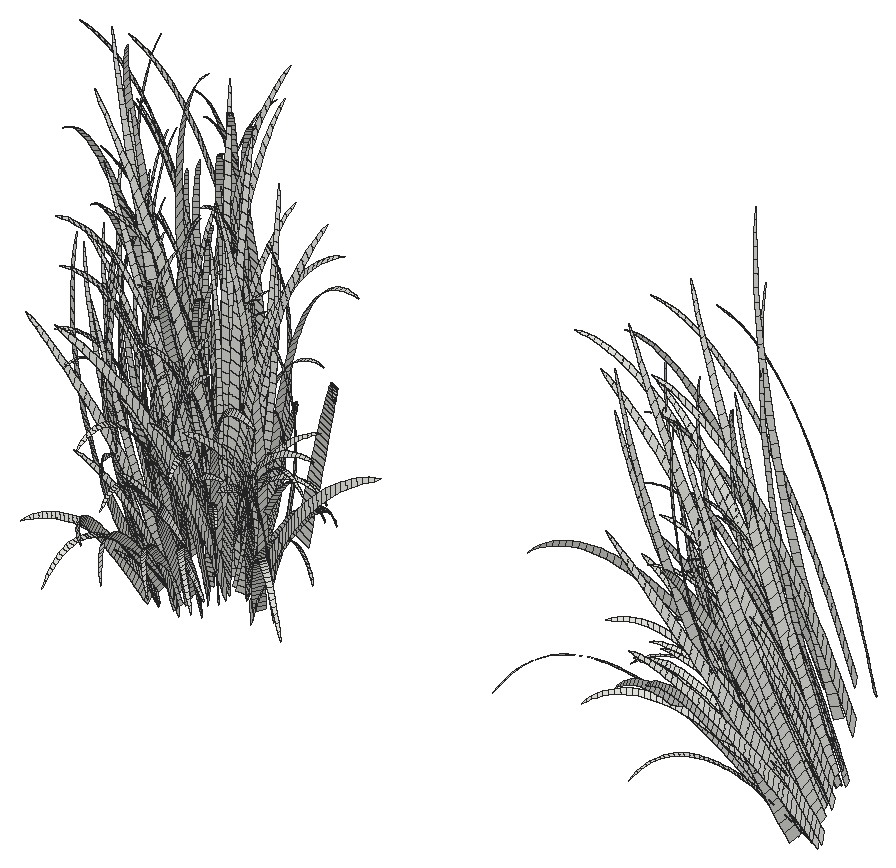
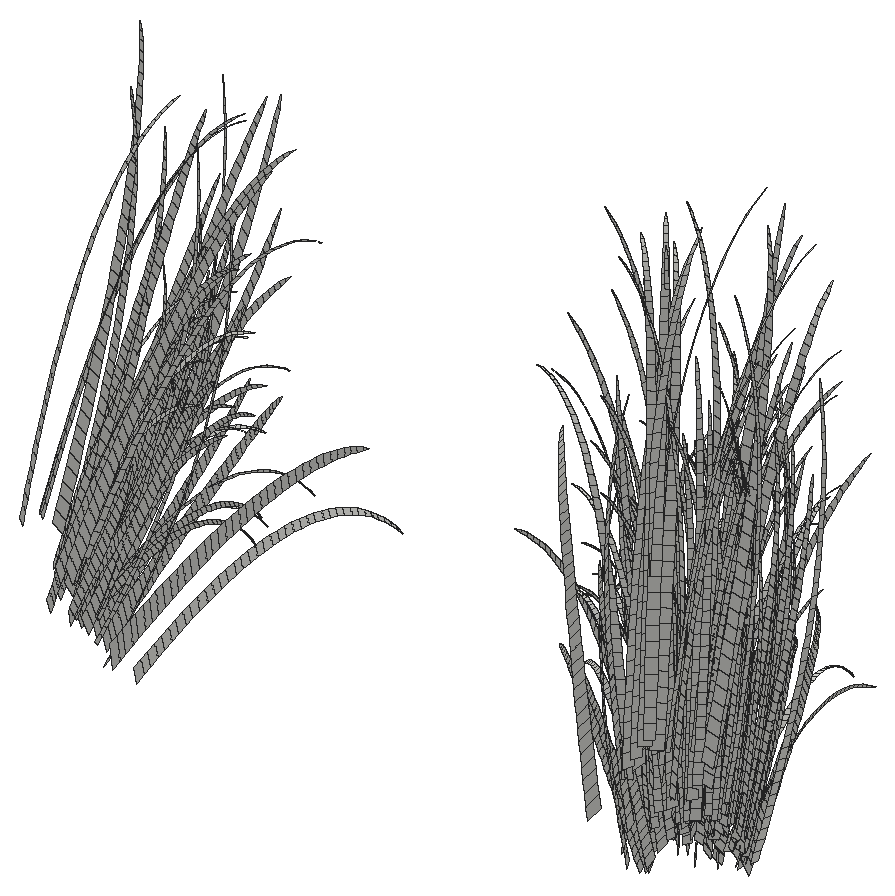
# SketchUp Ruby script. Lengths in inches.
U = 1.inch
M = Sketchup.active_model
def pt(a) = Geom::Point3d.new(a.map { |v| v * U })
def face(e, loops, mat)
  f = e.add_face(loops[0].map { |a| pt(a) })
  loops[1..].each { |l| e.add_face(l.map { |a| pt(a) }).erase! }
  f.material = f.back_material = mat if mat
  f
end
# faces: each face lists its corners as indices into pts; further lists are holes
def faces(e, pts, list, mat = nil) = list.each { |f| face(e, (f[0].is_a?(Array) ? f : [f]).map { |l| l.map { |i| pts[i] } }, mat) }
# xy, xz, yz: faces in a plane at the given z, y or x. An outline is a flat list of corners, or four numbers for a rectangle; further outlines are holes
def ring(l) = l.size == 4 ? [[l[0], l[1]], [l[2], l[1]], [l[2], l[3]], [l[0], l[3]]] : l.each_slice(2).to_a
def flat(e, list, mat, &to3) = list.each { |f| face(e, (f[0].is_a?(Array) ? f : [f]).map { |l| ring(l).map { |u, v| to3.(u, v) } }, mat) }
def xy(e, z, list, mat = nil) = flat(e, list, mat) { |x, y| [x, y, z] }
def xz(e, y, list, mat = nil) = flat(e, list, mat) { |x, z| [x, y, z] }
def yz(e, x, list, mat = nil) = flat(e, list, mat) { |y, z| [x, y, z] }
def lines(e, pts, list) = list.each { |a, b| e.add_line(pt(pts[a]), pt(pts[b])) }
# prism: a flat outline (further loops are holes) pulled along v
def prism(e, loops, v, mat = nil)
  f = face(e, loops, mat); d = Geom::Vector3d.new(v.map { |x| x * U })
  f.pushpull(f.normal.samedirection?(d) ? d.length : -d.length)
end
def box(e, o, s, mat = nil) = prism(e, [[o, [o[0] + s[0], o[1], o[2]], [o[0] + s[0], o[1] + s[1], o[2]], [o[0], o[1] + s[1], o[2]]]], [0, 0, s[2]], mat)
def at(x, y, z, deg = 0) = Geom::Transformation.translation(pt([x, y, z])) * Geom::Transformation.rotation(ORIGIN, Z_AXIS, deg.degrees)
def axes(o, x, y, z) = Geom::Transformation.new([*x, 0, *y, 0, *z, 0, *pt(o).to_a, 1])
def part(name) = M.definitions.add(name)
# library, detail: a bought-in or finely detailed component or shape, given as its bounding box
def library(name, o, s) = part(name).tap { |d| box(d.entities, o, s) }
def detail(e, o, s) = box(e.add_group.entities, o, s)
def put(e, d, t, mat = nil) = e.add_instance(d, t).tap { |i| i.material = mat if mat }
def group(e, t, mat = nil) = e.add_group.tap { |g| g.transformation = t; g.material = mat if mat }.entities
root = M.entities
c1 = part("fur_instance\#8")
p = [[-0.25,1.49,0.03],[0.25,-1.49,-0.03],[0.44,-1.47,1.51],[-0.05,1.47,1.57],[0.65,-1.44,3.05],[0.16,1.45,3.11],
  [0.86,-1.42,4.59],[0.38,1.44,4.65],[1.1,-1.39,6.13],[0.62,1.43,6.18],[1.34,-1.35,7.66],[0.875,1.42,7.72],
  [1.6,-1.32,9.19],[1.14,1.41,9.25],[1.88,-1.28,10.72],[1.43,1.41,10.78],[2.18,-1.24,12.25],[1.73,1.41,12.3],
  [2.49,-1.19,13.77],[2.05,1.41,13.82],[2.83,-1.15,15.29],[2.4,1.41,15.34],[3.18,-1.09,16.8],[2.76,1.42,16.85],
  [3.56,-1.03,18.31],[3.14,1.43,18.35],[3.96,-0.97,19.81],[3.55,1.44,19.85],[4.38,-0.91,21.3],[3.99,1.46,21.35],
  [4.84,-0.83,22.78],[4.45,1.48,22.83],[5.32,-0.76,24.26],[4.93,1.51,24.31],[5.82,-0.67,25.73],[5.45,1.54,25.77],
  [6.36,-0.59,27.18],[6,1.57,27.23],[6.93,-0.49,28.625],[6.58,1.61,28.67],[7.54,-0.39,30.05],[7.19,1.66,30.1],
  [8.18,-0.28,31.47],[7.84,1.71,31.51],[8.85,-0.16,32.86],[8.53,1.77,32.9],[9.57,-0.04,34.24],[9.25,1.83,34.27],
  [10.32,0.09,35.59],[10.02,1.9,35.625],[11.12,0.23,36.92],[10.82,1.97,36.95],[11.95,0.38,38.22],[11.67,2.06,38.25],
  [12.84,0.54,39.49],[12.57,2.14,39.52],[13.76,0.71,40.73],[13.51,2.24,40.76],[14.73,0.89,41.93],[14.49,2.34,41.95],
  [15.75,1.08,43.09],[15.52,2.45,43.11],[16.82,1.28,44.2],[16.6,2.5625,44.23],[17.93,1.5,45.27],[17.73,2.68,45.29],
  [19.08,1.73,46.28],[18.9,2.81,46.3],[20.29,1.97,47.24],[20.125,2.93,47.26],[21.53,2.22,48.13],[21.39,3.0625,48.15],
  [22.82,2.5,48.96],[22.7,3.1875,48.98],[24.14,2.8125,49.72],[24.06,3.3,49.73],[25.48,3.27,50.41]]
faces(c1.entities,p,[[0,1,2,3],[3,2,4,5],[5,4,6,7],[7,6,8,9],[9,8,10,11],[11,10,12,13],[13,12,14,15],[15,14,16,17],
  [17,16,18,19],[19,18,20,21],[21,20,22,23],[23,22,24,25],[25,24,26,27],[27,26,28,29],[29,28,30,31],[31,30,32,33],
  [33,32,34,35],[35,34,36,37],[37,36,38,39],[39,38,40,41],[41,40,42,43],[43,42,44,45],[45,44,46,47],[47,46,48,49],
  [49,48,50,51],[51,50,52,53],[53,52,54,55],[55,54,56,57],[57,56,58,59],[59,58,60,61],[61,60,62,63],[63,62,64,65],
  [65,64,66,67],[67,66,68,69],[69,68,70,71],[71,70,72,73],[73,72,74,75],[75,74,76]])
put(root,c1,axes([166.25,63.07,1.92],[-0.13424,-0.03889,-0.12787],[0.08866,-0.05443,-0.25596],[0.01839,-0.13945,0.22254]))
put(root,c1,axes([165.46,64.55,5.08],[0.0286,0.11518,0.18982],[-0.16763,0.04809,-0.0018],[-0.022,-0.10604,0.33361]))
put(root,c1,axes([164.88,64.7,4.7],[0.09089,0.09523,0.11248],[-0.12952,0.09997,0.00707],[-0.03129,-0.06837,0.34303]))
put(root,c1,axes([165.62,64.97,5.11],[0.0055,0.12915,0.11043],[-0.15799,0.02454,-0.01796],[-0.01431,-0.07554,0.33727]))
put(root,c1,axes([163.9,66.85,7.83],[0.2061,-0.01344,0.1131],[-0.02793,0.18662,0.09605],[-0.05077,-0.08252,0.4557]))
put(root,c1,axes([165.83,63.37,2.85],[-0.02267,0.09523,0.24051],[-0.16406,0.00552,-0.03477],[-0.00627,-0.12634,0.28034]))
put(root,c1,axes([164.71,65.7,5.77],[0.13539,0.06511,0.11886],[-0.10233,0.13809,0.02305],[-0.04143,-0.06734,0.37184]))
put(root,c1,axes([166.55,66.6,6.71],[-0.12883,-0.11449,0.01319],[0.1336,-0.12723,-0.04151],[0.01291,-0.04776,0.41418]))
put(root,c1,axes([164.98,66.85,9.62],[0.02992,-0.20268,-0.17218],[0.24479,0.00013,0.02509],[-0.00825,-0.12029,0.52424]))
put(root,c1,axes([166.57,67.86,7.57],[-0.11995,-0.14094,0.03187],[0.15995,-0.12378,-0.02155],[0.01135,-0.03745,0.44662]))
put(root,c1,axes([166.64,68.1,10.24],[-0.1863,-0.12854,0.00057],[0.15019,-0.16226,-0.16735],[0.0425,-0.10509,0.5177]))
put(root,c1,axes([166.15,66.31,6.08],[-0.07961,-0.13689,0.01423],[0.15313,-0.0843,-0.034],[0.01219,-0.0383,0.38556]))
put(root,c1,axes([166.14,66.73,6.48],[-0.07772,-0.14595,0.01956],[0.16231,-0.0838,-0.0308],[0.01178,-0.03674,0.40206]))
put(root,c1,axes([166.2,66.22,5.7],[-0.07124,-0.13476,0.02236],[0.14958,-0.07747,-0.02272],[0.00941,-0.03103,0.37011]))
put(root,c1,axes([165.92,63.66,3.64],[0.01737,0.09262,0.24572],[-0.16736,0.02852,0.02395],[-0.00637,-0.12835,0.28481]))
put(root,c1,axes([164.29,67.91,10.27],[0.18706,-0.15692,-0.05371],[0.1539,0.13296,0.16341],[-0.03534,-0.11123,0.5203]))
put(root,c1,axes([165.04,64.9375,4.9],[0.13738,0.0414,0.0972],[-0.07592,0.13055,0.05523],[-0.03104,-0.06782,0.34028]))
put(root,c1,axes([166.43,64.96,6.06],[-0.07914,0.12591,0.21103],[-0.17333,-0.05924,-0.02394],[0.02804,-0.12033,0.37519]))
put(root,c1,axes([166.53,64.61,5.43],[-0.10701,-0.11213,-0.12442],[0.15233,-0.07687,-0.16606],[0.02739,-0.11756,0.36656]))
put(root,c1,axes([167.18,64.56,4.8],[-0.16995,0.00239,0.1052],[-0.0155,-0.13112,-0.16118],[0.04006,-0.1041,0.34197]))
put(root,c1,axes([165.02,63.27,2.44],[0.11054,0.06076,0.32124],[-0.18174,0.06569,0.1961],[-0.00805,-0.18258,0.29226]))
put(root,c1,axes([165.52,66.46,8.02],[0.04164,-0.17352,-0.14577],[0.20763,0.01338,0.03275],[-0.00709,-0.10329,0.45016]))
put(root,c1,axes([165.47,63.36,2.71],[0.07036,0.07691,0.22077],[-0.15002,0.05652,0.10186],[-0.00627,-0.1264,0.28049]))
put(root,c1,axes([165.04,65.46,6.11],[0.15043,0.06237,0.10618],[-0.10193,0.14112,0.07332],[-0.02651,-0.08344,0.39031]))
put(root,c1,axes([165.12,64.57,4.85],[0.1599,-0.01285,0.09328],[-0.0299,0.12534,0.15874],[-0.03604,-0.09723,0.32437]))
put(root,c1,axes([167.45,63.47,2.95],[-0.19796,-0.00213,0.19119],[-0.0584,-0.09827,-0.32515],[0.05556,-0.17894,0.29438]))
put(root,c1,axes([165.96,64.5,5.42],[-0.00485,-0.13574,-0.20923],[0.19174,-0.01245,-0.03687],[0.01079,-0.12284,0.3739]))
put(root,c1,axes([164.93,64.14,4.3],[0.16477,0.01322,0.09468],[-0.05646,0.12716,0.16983],[-0.02254,-0.10862,0.34171]))
put(root,c1,axes([167.59,66.57,6.59],[-0.18521,-0.02955,0.11381],[0.03239,-0.17376,-0.06029],[0.05035,-0.05919,0.41626]))
put(root,c1,axes([167.33,64.2,3.87],[-0.14955,-0.02951,0.08847],[0.01953,-0.12021,-0.14832],[0.04773,-0.08667,0.30915]))
put(root,c1,axes([165.31,63.6,3.27],[0.16669,-0.01734,0.08094],[-0.02966,0.10281,0.23812],[-0.02771,-0.12642,0.29024]))
put(root,c1,axes([165.51,63.39,2.97],[0.12347,0.06755,0.21237],[-0.14396,0.08585,0.17984],[-0.00718,-0.14468,0.32104]))
put(root,c1,axes([167.49,65.25,6.875],[-0.16708,-0.12567,-0.06302],[0.15179,-0.11958,-0.24667],[0.05298,-0.1377,0.45233]))
put(root,c1,axes([165.61,67.21,6.375],[0.10751,-0.14401,0.02773],[0.14274,0.0886,-0.01156],[-0.00773,-0.0245,0.39927]))
put(root,c1,axes([166.7,63.22,2.44],[-0.04322,-0.08103,-0.33227],[0.19342,-0.01502,-0.11763],[0.02265,-0.17179,0.27415]))
put(root,c1,axes([166.97,66.19,5.24],[-0.08777,-0.12311,0.07978],[0.13105,-0.09185,-0.0647],[0.04014,-0.02395,0.34954]))
put(root,c1,axes([167.5,64.67,5.74],[-0.14817,-0.12463,-0.07303],[0.15181,-0.10509,-0.22784],[0.04979,-0.1294,0.42509]))
put(root,c1,axes([165.78,64.26,4.62],[0.12885,0.05972,0.11755],[-0.10424,0.10176,0.1411],[-0.00603,-0.1057,0.32265]))
put(root,c1,axes([167.44,63.19,1.56],[-0.14554,-0.04613,0.08103],[0.01279,-0.07284,-0.26823],[0.06295,-0.12513,0.21981]))
put(root,c1,axes([167.69,64.25,4.59],[-0.14966,0.06135,0.2769],[-0.12806,-0.11932,-0.12286],[0.06613,-0.14624,0.35295]))
put(root,c1,axes([167.44,63.18,1.64],[-0.08929,0.05587,0.30832],[-0.15159,-0.06244,-0.09121],[0.04736,-0.15254,0.25094]))
put(root,c1,axes([165.61,65.71,5.67],[0.16373,-0.03857,0.00921],[0.02397,0.14494,0.04432],[-0.01107,-0.05099,0.36849]))
put(root,c1,axes([166.875,65.56,5.39],[-0.04201,-0.14205,-0.02716],[0.15521,-0.03808,-0.10788],[0.03986,-0.0584,0.35377]))
put(root,c1,axes([165.8,63.04,1.76],[0.15269,-0.07243,-0.24019],[0.13551,0.04613,0.26977],[-0.00773,-0.17522,0.28049]))
put(root,c1,axes([165.85,64.98,5.3],[0.14874,-0.07113,-0.04632],[0.06911,0.1145,0.10604],[-0.00549,-0.08,0.34865]))
put(root,c1,axes([167.69,65.57,4.8],[-0.14662,-0.03521,0.15792],[0.02351,-0.14317,-0.07806],[0.07228,-0.05609,0.32502]))
put(root,c1,axes([165.73,66.05,6.11],[0.16142,-0.07143,-0.01571],[0.0631,0.13884,0.04506],[-0.00507,-0.05525,0.3852]))
put(root,c1,axes([165.76,67.26,7.48],[0.12208,-0.15013,-0.02869],[0.15272,0.10311,-0.03034],[0.01381,-0.04339,0.43679]))
put(root,c1,axes([167.9375,64.5625,5.75],[-0.10088,0.13062,0.3695],[-0.228,-0.07812,-0.04804],[0.0527,-0.18996,0.43195]))
put(root,c1,axes([166.04,63,1.69],[0.1143,0.07759,0.29786],[-0.18253,0.04472,0.24081],[0.02462,-0.18668,0.29791]))
put(root,c1,axes([166.21,65.15,6.22],[0.10618,-0.13596,-0.12929],[0.15853,0.08066,0.0353],[0.01505,-0.09183,0.40695]))
put(root,c1,axes([167.32,64.25,4.92],[-0.04153,-0.12718,-0.27595],[0.20481,-0.00989,-0.14624],[0.04417,-0.15922,0.36205]))
put(root,c1,axes([165.9,63.21,2.53],[0.19045,-0.03751,-0.06848],[0.03839,0.07261,0.33686],[-0.00736,-0.16676,0.26694]))
put(root,c1,axes([166.48,65.09,5.64],[0.0987,0.11897,0.05521],[-0.14378,0.08662,0.10909],[0.02282,-0.08103,0.37425]))
put(root,c1,axes([166.45,66.72,5.8],[0.11708,-0.12342,-0.00631],[0.12225,0.10057,-0.03033],[0.0076,-0.02912,0.37804]))
put(root,c1,axes([166.43,63.2,2.43],[0.10158,-0.06914,-0.32205],[0.1701,0.0448,0.14301],[0.02265,-0.17174,0.27406]))
put(root,c1,axes([167.35,63.58,3.05],[0.00165,-0.10984,-0.26082],[0.18149,0.01453,-0.07449],[0.03836,-0.13829,0.31445]))
put(root,c1,axes([168.66,65.85,6.76],[-0.1604,-0.13739,-0.02167],[0.15059,-0.11716,-0.25101],[0.06963,-0.12643,0.45099]))
put(root,c1,axes([169.34,64.98,5.43],[-0.21667,0.03837,0.29524],[-0.10928,-0.16078,-0.2283],[0.08148,-0.18018,0.43484]))
put(root,c1,axes([166.38,63.9,3.98],[0.15315,-0.04031,-0.07636],[0.04669,0.1064,0.16007],[0.009,-0.10254,0.31211]))
put(root,c1,axes([168.81,64.41,3.65],[-0.18644,-0.03104,0.19118],[-0.0143,-0.14214,-0.22961],[0.08573,-0.13206,0.3504]))
put(root,c1,axes([167.14,65.08,5.45],[0.0438,-0.14683,-0.11127],[0.16937,0.03664,-0.05087],[0.03107,-0.07683,0.37846]))
put(root,c1,axes([168.82,67.99,9.95],[-0.20857,-0.13075,0.08955],[0.12369,-0.16885,-0.26752],[0.09431,-0.12712,0.50956]))
put(root,c1,axes([166.66,65.82,5.36],[0.13914,-0.08385,-0.03496],[0.08075,0.12335,-0.00894],[0.01158,-0.03859,0.35924]))
put(root,c1,axes([168.38,63.78,1.59],[-0.12758,-0.07753,0.0557],[0.04435,-0.06394,-0.27127],[0.08127,-0.11212,0.2187]))
put(root,c1,axes([168.66,64.0625,2.3],[-0.14977,-0.06071,0.14936],[0.00439,-0.0935,-0.26844],[0.09015,-0.12438,0.2426]))
put(root,c1,axes([168.03,64.36,3.39],[-0.08522,-0.11751,-0.02593],[0.11177,-0.04315,-0.23298],[0.08081,-0.09116,0.27707]))
put(root,c1,axes([166.82,63.84,3.77],[0.12624,-0.07118,-0.14847],[0.09892,0.09301,0.09957],[0.0236,-0.10128,0.3158]))
put(root,c1,axes([166.64,65.81,6.13],[0.11075,-0.11944,-0.11937],[0.13443,0.0987,-0.0216],[0.03784,-0.07056,0.38011]))
put(root,c1,axes([165.875,66.85,9.9],[0.24074,-0.08114,-0.0797],[0.07823,0.19128,0.15934],[0.00596,-0.12377,0.53808]))
put(root,c1,axes([169.67,64.16,3.13],[-0.23798,-0.07441,0.13592],[0.01899,-0.11962,-0.43721],[0.10286,-0.20447,0.35918]))
put(root,c1,axes([168.3,64.73,3.57],[-0.09743,0.06774,0.23139],[-0.09599,-0.11967,0.05358],[0.09249,-0.07723,0.28321]))
put(root,c1,axes([167.95,64.89,5.37],[-0.02184,-0.15888,-0.15748],[0.19236,-0.00034,-0.15603],[0.06127,-0.11125,0.39683]))
put(root,c1,axes([166.74,65.52,5.3125],[0.15222,0.03642,-0.07852],[-0.03946,0.13914,0.07531],[0.03898,-0.05711,0.34597]))
put(root,c1,axes([168.65,65.35,3.41],[-0.11286,0.04976,0.22948],[-0.06771,-0.13658,0.05175],[0.0986,-0.05954,0.28318]))
put(root,c1,axes([167.36,66.85,6.28],[0.07494,-0.15978,-0.03962],[0.16264,0.06715,-0.11216],[0.04856,-0.037,0.39794]))
put(root,c1,axes([168.7,65.16,4.61],[-0.12334,-0.12969,0.01714],[0.11431,-0.07492,-0.27994],[0.09668,-0.10907,0.33149]))
put(root,c1,axes([167.19,63.32,2.45],[0.09702,-0.05494,-0.31246],[0.152,0.06601,0.10474],[0.04854,-0.15634,0.25719]))
put(root,c1,axes([168.33,68.49,9.47],[-0.02329,-0.21903,-0.03429],[0.23378,-0.02287,-0.15724],[0.06291,-0.07396,0.52011]))
put(root,c1,axes([167.12,66.1,4.98],[0.13682,-0.07692,-0.07129],[0.07213,0.1295,-0.07116],[0.03936,-0.02349,0.34277]))
put(root,c1,axes([166.67,63.61,3.85],[0.22137,0.04305,0.07377],[-0.08148,0.12835,0.33894],[0.02049,-0.18118,0.40078]))
put(root,c1,axes([167.07,63.89,3.92],[0.16263,0.05278,0.0273],[-0.0671,0.09353,0.2615],[0.03718,-0.13404,0.3048]))
put(root,c1,axes([166.95,66.0625,5.73],[0.1463,-0.07615,-0.10409],[0.07711,0.13848,-0.04067],[0.04559,-0.04329,0.3674]))
put(root,c1,axes([169.1,66.03,4.17],[-0.14023,0.01888,0.26296],[-0.04453,-0.1614,-0.00292],[0.11023,-0.06656,0.31656]))
put(root,c1,axes([168.97,64.38,2.35],[-0.13012,-0.10057,0.10963],[0.04873,-0.08061,-0.28847],[0.10836,-0.10823,0.24566]))
put(root,c1,axes([167.54,65.97,5.05],[0.10839,-0.11453,-0.08174],[0.11795,0.10157,-0.07097],[0.04416,-0.04194,0.35588]))
put(root,c1,axes([167.34,65.1,6.95],[0.14666,-0.13638,-0.25039],[0.18844,0.10867,0.09026],[0.03514,-0.1508,0.47019]))
put(root,c1,axes([169.375,66.26,4],[-0.14894,-0.04461,0.24591],[0.01234,-0.15892,-0.10432],[0.11196,-0.06761,0.32156]))
put(root,c1,axes([168.92,68.4,8.6875],[-0.02212,-0.21398,-0.03391],[0.22838,-0.02174,-0.15347],[0.06144,-0.07223,0.50797]))
put(root,c1,axes([166.89,66.9,9.03],[0.23315,0.01342,-0.06471],[-0.02237,0.19719,0.15093],[0.03065,-0.10883,0.50265]))
put(root,c1,axes([167.65,65.17,4.86],[0.10539,0.11766,-0.04264],[-0.11395,0.08648,0.1779],[0.06944,-0.07112,0.33381]))
put(root,c1,axes([169.58,65.09,3.33],[-0.10089,0.09227,0.28247],[-0.13958,-0.12254,0.05217],[0.09902,-0.11171,0.33951]))
put(root,c1,axes([168.98,65.4,5.95],[-0.03936,0.14543,0.30601],[-0.20696,-0.07562,0.14027],[0.09659,-0.14879,0.39477]))
put(root,c1,axes([167.26,63.79,3.74],[0.19476,0.01919,-0.07142],[-0.00771,0.11743,0.2824],[0.0412,-0.14851,0.33769]))
put(root,c1,axes([167.72,68.37,10.66],[0.12423,-0.19532,-0.16493],[0.21975,0.1108,-0.06089],[0.05484,-0.10226,0.55089]))
put(root,c1,axes([168.03,65.86,7.06],[0.10368,0.16194,0.09463],[-0.18699,0.06759,0.22582],[0.06767,-0.12287,0.43828]))
put(root,c1,axes([167.83,63.51,2.01],[0.10797,-0.02278,-0.25368],[0.09924,0.08349,0.12145],[0.06318,-0.1256,0.22064]))
put(root,c1,axes([167.71,64.28,4.37],[0.12346,-0.06874,-0.2664],[0.133,0.10274,0.08323],[0.06093,-0.13474,0.32518]))
put(root,c1,axes([168.8,67.7,8.47],[-0.03736,-0.20284,-0.08426],[0.21276,-0.01244,-0.24024],[0.09664,-0.09898,0.46456]))
put(root,c1,axes([167.92,67.38,9.57],[0.143,-0.17445,-0.17187],[0.20045,0.12222,-0.01071],[0.04373,-0.10813,0.53269]))
put(root,c1,axes([167.67,63.54,2.48],[0.15494,0.00054,-0.15254],[0.03594,0.10834,0.19122],[0.0534,-0.11809,0.285]))
put(root,c1,axes([167.98,65.4,5.71],[0.10826,0.14171,0.01778],[-0.14869,0.07846,0.21324],[0.07154,-0.09642,0.38649]))
put(root,c1,axes([168.65,64.39,3.98],[0.01148,-0.14011,-0.26001],[0.19146,0.05137,-0.16224],[0.08794,-0.13547,0.35942]))
put(root,c1,axes([168.43,64.33,2.75],[0.05454,-0.09644,-0.21571],[0.13016,0.08062,-0.0942],[0.08114,-0.09154,0.27821]))
put(root,c1,axes([167.8,68.5,10.35],[0.15717,-0.16888,-0.16909],[0.19008,0.14007,-0.03029],[0.05359,-0.09991,0.53827]))
put(root,c1,axes([169.71,65.53,3.6875],[-0.06239,0.13265,0.23168],[-0.15342,-0.10065,0.1704],[0.112,-0.09352,0.34293]))
put(root,c1,axes([169.36,67.65,4.85],[-0.06465,-0.16754,0.157],[0.14103,-0.07728,-0.22676],[0.11827,-0.02606,0.33858]))
put(root,c1,axes([167.54,63.45,2.92],[0.19478,-0.02841,-0.30734],[0.1247,0.10642,0.29017],[0.06226,-0.20052,0.32988]))
put(root,c1,axes([168.1875,63.57,2.52],[0.10305,-0.05896,-0.3685],[0.16571,0.09891,0.06527],[0.08407,-0.16713,0.29358]))
put(root,c1,axes([168.05,66.04,8.22],[0.19083,0.13184,0.05677],[-0.15811,0.13743,0.27367],[0.05817,-0.15117,0.49659]))
put(root,c1,axes([168.51,65.21,4.67],[0.13121,0.11551,-0.02739],[-0.11587,0.10209,0.2018],[0.06808,-0.09176,0.36783]))
put(root,c1,axes([168.79,66.79,2.6],[0.04832,-0.14518,0.00787],[0.12065,0.04323,-0.22286],[0.09094,-0.00311,0.27632]))
put(root,c1,axes([169.64,64.8125,4.04],[-0.00332,0.15612,0.27725],[-0.2105,-0.04955,0.19049],[0.09652,-0.14869,0.3945]))
put(root,c1,axes([168.76,65.87,3.07],[0.0496,-0.12974,-0.10453],[0.11629,0.07093,-0.20268],[0.09864,-0.03996,0.27723]))
put(root,c1,axes([169.31,66.11,1.875],[-0.03175,-0.14429,0.13902],[0.10175,-0.04851,-0.23869],[0.11949,-0.01479,0.22844]))
put(root,c1,axes([169.65,65.14,2.65],[-0.05491,0.09737,0.28251],[-0.12379,-0.11722,0.16383],[0.12913,-0.0934,0.26231]))
put(root,c1,axes([169.85,65.13,2.47],[-0.0662,0.08995,0.30205],[-0.12202,-0.12772,0.14438],[0.13238,-0.09575,0.2689]))
put(root,c1,axes([170.78,65.6,3.46],[-0.14869,0.01051,0.38769],[-0.10168,-0.16677,-0.09879],[0.14048,-0.14032,0.31849]))
put(root,c1,axes([168.63,64.83,2.98],[0.12216,0.08749,-0.1288],[-0.05725,0.10364,0.19567],[0.09123,-0.07618,0.27934]))
put(root,c1,axes([169.91,65.27,2.55],[-0.06626,-0.1567,-0.04431],[0.12258,-0.00555,-0.33309],[0.13287,-0.09611,0.2699]))
put(root,c1,axes([170.18,66.85,2.07],[-0.09134,-0.12785,0.22656],[0.07697,-0.11104,-0.22116],[0.1384,-0.04262,0.25929]))
put(root,c1,axes([169.37,64.43,2.89],[0.07572,0.13089,0.20219],[-0.15985,-0.01369,0.30106],[0.10643,-0.14683,0.2864]))
put(root,c1,axes([168.76,66.13,5.26],[0.16409,-0.04331,-0.20606],[0.05728,0.16704,-0.00737],[0.08461,-0.06565,0.38043]))
put(root,c1,axes([169.17,66.375,2.1],[0.06266,-0.1249,-0.10853],[0.0861,0.08678,-0.25374],[0.11938,-0.01478,0.22823]))
put(root,c1,axes([168.95,64.99,3.17],[0.14109,0.00407,-0.23949],[0.03377,0.14579,0.07817],[0.0981,-0.08192,0.30039]))
put(root,c1,axes([169.21,65.55,3.76],[0.12005,-0.06141,-0.26447],[0.09556,0.14151,-0.0324],[0.10376,-0.08664,0.31771]))
put(root,c1,axes([169.08,64.79,3.4],[0.16454,0.02683,-0.22071],[0.01929,0.1451,0.16624],[0.09525,-0.10745,0.32659]))
put(root,c1,axes([171.61,65.3,2.04],[-0.15559,-0.16713,0.03304],[0.11706,-0.06849,-0.43118],[0.15185,-0.15167,0.34426]))
put(root,c1,axes([169.54,66.41,2.01],[0.068,-0.12804,-0.12081],[0.08818,0.09434,-0.26208],[0.12484,-0.01545,0.23865]))
put(root,c1,axes([168.99,66.45,6.79],[0.20769,0.04966,-0.15926],[-0.03101,0.17814,0.18526],[0.08167,-0.11008,0.44127]))
put(root,c1,axes([169.58,65.6,2.42],[0.06859,-0.09014,-0.25373],[0.09618,0.12505,-0.16822],[0.12923,-0.06487,0.24688]))
put(root,c1,axes([169.1,64.54,4.58],[0.20792,-0.04098,-0.29203],[0.11115,0.15527,0.21492],[0.07916,-0.17504,0.42246]))
put(root,c1,axes([169.625,65.61,2.97],[0.12063,-0.06515,-0.25144],[0.08341,0.14829,-0.07405],[0.10987,-0.06634,0.31554]))
put(root,c1,axes([169.8,65.05,4.63],[0.15805,0.15051,0.05502],[-0.15454,0.08321,0.34889],[0.10135,-0.15612,0.41421]))
put(root,c1,axes([169.93,67.2,7.15],[0.20327,-0.05604,-0.25675],[0.08292,0.19878,0.03195],[0.09822,-0.10059,0.47212]))
put(root,c1,axes([171.2,64.87,2.04],[0.10396,-0.07911,-0.43973],[0.18772,0.13868,-0.01375],[0.12911,-0.17813,0.34745]))
put(root,c1,axes([171.59,67.78,4.82],[0.04979,-0.1895,-0.18773],[0.18438,0.09265,-0.2851],[0.14308,-0.0864,0.41092]))
put(root,c1,axes([170.6875,64.82,1.74],[0.1674,0.12348,-0.15342],[-0.05527,0.10723,0.36025],[0.13749,-0.13733,0.3117]))
put(root,c1,axes([201.4,68.76,3.75],[-0.02161,-0.16628,-0.28389],[0.16425,-0.14433,0.32408],[-0.18224,-0.08282,0.344]))
put(root,c1,axes([201.46,66.78,1.77],[-0.07933,-0.07892,-0.44402],[0.19255,-0.17562,0.06989],[-0.14788,-0.14983,0.35337]))
put(root,c1,axes([204.14,67.33,7.77],[-0.23554,0.05296,-0.19778],[0.0198,-0.2043,-0.19606],[-0.09324,-0.11985,0.49597]))
put(root,c1,axes([203.9375,68.95,7.54],[-0.04128,-0.19919,-0.10991],[0.2038,-0.09544,0.23105],[-0.11682,-0.05581,0.46862]))
put(root,c1,axes([203.11,67.08,2],[0.13283,-0.0342,0.36955],[-0.05695,0.18902,0.06859],[-0.15898,-0.07225,0.3001]))
put(root,c1,axes([206.08,64.83,2.51],[-0.12873,0.10197,-0.18861],[-0.01018,-0.10343,-0.24101],[-0.11719,-0.08155,0.24232]))
put(root,c1,axes([205.35,68.05,6.68],[-0.08516,-0.14739,-0.15062],[0.16457,-0.13044,0.17116],[-0.1041,-0.04973,0.41758]))
put(root,c1,axes([206.17,64.22,2.92],[-0.15935,0.03269,-0.28558],[0.09029,-0.13292,-0.22683],[-0.09601,-0.14239,0.28508]))
put(root,c1,axes([206.17,64.65,2.21],[-0.14081,0.09765,-0.1356],[-0.01218,-0.08683,-0.27326],[-0.10036,-0.10168,0.23982]))
put(root,c1,axes([206.3125,66.09,6.5],[-0.18347,0.1171,-0.07334],[-0.07461,-0.13251,-0.22152],[-0.07812,-0.10043,0.41558]))
put(root,c1,axes([206.19,64.51,2.71],[-0.15082,0.11254,-0.07354],[-0.05779,-0.09193,-0.25822],[-0.08893,-0.09949,0.31347]))
put(root,c1,axes([206.18,66.52,5.94],[-0.149,-0.04647,-0.21352],[0.09287,-0.17245,0.02054],[-0.09229,-0.06322,0.38876]))
put(root,c1,axes([205.69,64.27,3.03],[-0.09966,0.12678,0.30336],[-0.19172,0.0268,-0.26785],[-0.07616,-0.17634,0.31506]))
put(root,c1,axes([204.9375,66.42,3.22],[0.05365,-0.16969,-0.03778],[0.13986,-0.00916,0.27148],[-0.1167,-0.06341,0.32492]))
put(root,c1,axes([206.4,64.77,2.88],[-0.10552,0.13111,0.03774],[-0.1075,-0.03434,-0.24755],[-0.08294,-0.09279,0.29236]))
put(root,c1,axes([206.95,64.85,6.41],[-0.23362,0.09843,0.07428],[-0.08627,-0.11761,-0.36241],[-0.04076,-0.18596,0.42692]))
put(root,c1,axes([206.14,65.09,2.59],[-0.05906,0.14196,0.06951],[-0.12604,0.00717,-0.23329],[-0.09379,-0.07416,0.28621]))
put(root,c1,axes([204.84,65.05,1.76],[0.08197,-0.14846,-0.17255],[0.1435,-0.03613,0.3122],[-0.11735,-0.1189,0.28043]))
put(root,c1,axes([206.97,67.41,9.42],[-0.2227,-0.02851,-0.13015],[0.07795,-0.20389,-0.10631],[-0.04666,-0.10194,0.51151]))
put(root,c1,axes([206.37,65.87,2.94],[-0.05395,-0.10392,-0.15053],[0.10796,-0.10426,0.17042],[-0.10255,-0.03484,0.272]))
put(root,c1,axes([206.95,64.13,3.64],[-0.17727,0.00029,-0.20455],[0.08516,-0.1353,-0.21935],[-0.05731,-0.14134,0.34686]))
put(root,c1,axes([206.71,64.61,3.51],[-0.10062,-0.049,-0.26041],[0.12035,-0.13237,-0.01381],[-0.08638,-0.09663,0.30447]))
put(root,c1,axes([207.01,66.22,4.12],[-0.12457,-0.03797,-0.15408],[0.05979,-0.14532,0.07008],[-0.07901,-0.02356,0.31353]))
put(root,c1,axes([206.65,64.01,4.09],[-0.15374,0.14658,0.25603],[-0.19784,-0.04817,-0.27014],[-0.04101,-0.18709,0.42951]))
put(root,c1,axes([205.05,65.41,1.76],[0.13307,-0.06357,0.27984],[-0.03809,0.14212,0.17121],[-0.12562,-0.08741,0.25976]))
put(root,c1,axes([206.92,64.3,2.375],[-0.0986,0.1202,0.03133],[-0.09749,-0.03341,-0.22837],[-0.07635,-0.08541,0.26912]))
put(root,c1,axes([206.71,64.0625,1.98],[-0.08725,-0.02366,-0.29756],[0.12591,-0.11202,-0.06714],[-0.0803,-0.1191,0.23844]))
put(root,c1,axes([207.24,64.14,2.95],[-0.15103,0.03829,-0.1475],[0.02836,-0.11444,-0.19385],[-0.06472,-0.10394,0.28282]))
put(root,c1,axes([204.54,65.9,3.56],[0.17403,-0.06722,0.24815],[-0.01797,0.16553,0.179],[-0.11789,-0.09322,0.35975]))
put(root,c1,axes([206.21,63.5625,1.96],[-0.07738,0.12181,0.42116],[-0.24475,0.02807,-0.19007],[-0.04925,-0.2161,0.35893]))
put(root,c1,axes([207.43,63.58,2.95],[-0.19758,0.0885,0.1271],[-0.09447,-0.05952,-0.37318],[-0.04202,-0.18438,0.30623]))
put(root,c1,axes([205.91,65.45,3.43],[0.04667,0.10587,0.22641],[-0.14224,0.11026,-0.13144],[-0.10087,-0.07976,0.30781]))
put(root,c1,axes([206.8,65,6.18],[-0.12023,0.16893,0.15811],[-0.19192,-0.04724,-0.20175],[-0.05017,-0.13536,0.45159]))
put(root,c1,axes([207.07,64.82,4.52],[-0.1513,-0.02821,-0.17374],[0.08683,-0.1419,-0.10144],[-0.05423,-0.09755,0.35603]))
put(root,c1,axes([207.18,64.62,3.44],[-0.07947,0.12548,0.07397],[-0.11521,-0.01055,-0.22059],[-0.07706,-0.08621,0.27164]))
put(root,c1,axes([206.89,66.85,3.86],[-0.06439,-0.12354,-0.04587],[0.12333,-0.08786,0.16125],[-0.07712,-0.0102,0.31415]))
put(root,c1,axes([206.34,65.11,2.49],[0.02731,-0.14018,-0.06519],[0.12315,-0.02871,0.2214],[-0.09827,-0.0534,0.27359]))
put(root,c1,axes([205.73,64.66,1.89],[0.09631,-0.13966,-0.10726],[0.11682,-0.00954,0.30869],[-0.10751,-0.10893,0.25692]))
put(root,c1,axes([207.66,64.74,5.09],[-0.18173,0.02045,-0.09763],[0.0261,-0.14072,-0.18343],[-0.04068,-0.10974,0.36609]))
put(root,c1,axes([206.14,65.89,3.28],[0.06905,-0.15041,0.07394],[0.1069,0.0384,0.22809],[-0.10814,-0.03674,0.28683]))
put(root,c1,axes([206.11,66.28,4.85],[0.02994,-0.16585,-0.05499],[0.16129,-0.01842,0.19273],[-0.08623,-0.05907,0.36324]))
put(root,c1,axes([207.75,63.5,2.53],[-0.18497,0.04944,-0.02341],[-0.00878,-0.07542,-0.33252],[-0.03553,-0.1559,0.25894]))
put(root,c1,axes([207.47,65.75,5.45],[-0.14413,-0.05167,-0.11933],[0.08701,-0.14734,-0.01287],[-0.04763,-0.0596,0.37283]))
put(root,c1,axes([207.18,63.85,2.15],[-0.04193,0.09854,0.23039],[-0.14173,0.04993,-0.18317],[-0.07748,-0.11492,0.23007]))
put(root,c1,axes([206.95,66.04,4.19],[-0.02354,-0.13666,-0.06934],[0.13862,-0.06024,0.1585],[-0.07899,-0.03774,0.31687]))
put(root,c1,axes([207.91,63.625,2.59],[-0.15528,0.03655,-0.09389],[0.01601,-0.10098,-0.21878],[-0.04549,-0.11219,0.27533]))
put(root,c1,axes([207.9375,64.46,4.13],[-0.15238,0.03287,-0.097],[0.00948,-0.12228,-0.14695],[-0.04746,-0.08538,0.3116]))
put(root,c1,axes([207.18,65.7,4.59],[-0.02967,-0.13006,-0.11002],[0.14258,-0.07093,0.13984],[-0.07655,-0.05244,0.32247]))
put(root,c1,axes([206.06,65.01,2.95],[0.10962,-0.14134,0.02858],[0.09848,0.05163,0.25611],[-0.09929,-0.07851,0.30299]))
put(root,c1,axes([207.55,65.02,5.3],[-0.07622,0.14548,0.11566],[-0.15943,-0.01772,-0.1678],[-0.05494,-0.09882,0.36066]))
put(root,c1,axes([208.28,65.69,8.0625],[-0.23536,0.00031,-0.04255],[0.03502,-0.16941,-0.26023],[-0.00865,-0.15175,0.46324]))
put(root,c1,axes([206.65,63.92,2.05],[0.07176,0.04443,0.32956],[-0.1495,0.11571,0.02095],[-0.08693,-0.12893,0.25813]))
put(root,c1,axes([207.8,67.92,8.8],[-0.16552,-0.11118,-0.05649],[0.14207,-0.16762,-0.00154],[-0.02412,-0.05905,0.48802]))
put(root,c1,axes([207.76,63.68,3.4],[-0.1192,0.12425,0.22535],[-0.17166,-0.03356,-0.21354],[-0.0342,-0.15606,0.35826]))
put(root,c1,axes([207.47,65.45,4.62],[-0.02927,-0.12714,-0.10789],[0.13946,-0.06963,0.13664],[-0.0749,-0.05131,0.31553]))
put(root,c1,axes([205.72,64.84,4.17],[0.13498,-0.15634,-0.12045],[0.15269,0.03421,0.29976],[-0.08583,-0.13785,0.37509]))
put(root,c1,axes([206.96,66.07,7.93],[-0.00008,0.17023,0.2439],[-0.22913,0.05018,-0.08813],[-0.05076,-0.13695,0.4569]))
put(root,c1,axes([205.79,66.21,5.49],[0.15632,-0.13539,0.07566],[0.09629,0.11232,0.20743],[-0.0859,-0.08088,0.3964]))
put(root,c1,axes([205.68,63.875,2.16],[0.17581,0.00429,0.35889],[-0.15371,0.13999,0.25001],[-0.08231,-0.1906,0.34052]))
put(root,c1,axes([206.87,65.44,6.28],[0.05112,0.14176,0.22694],[-0.19757,0.09246,-0.06236],[-0.06344,-0.11412,0.4165]))
